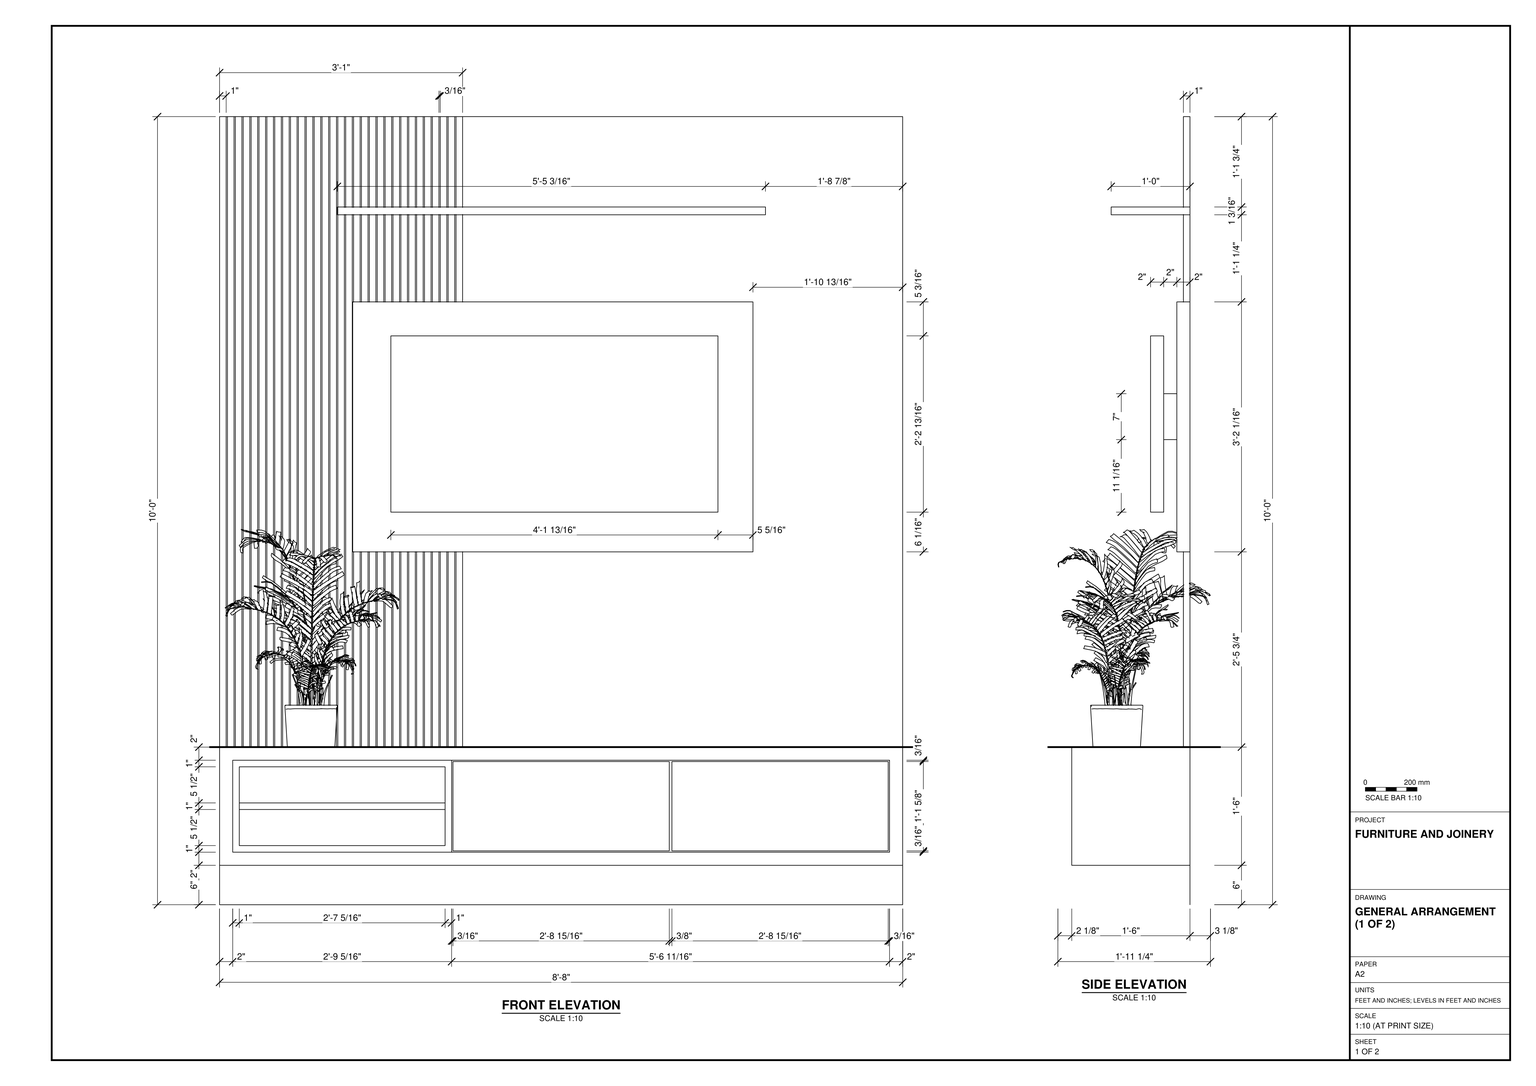
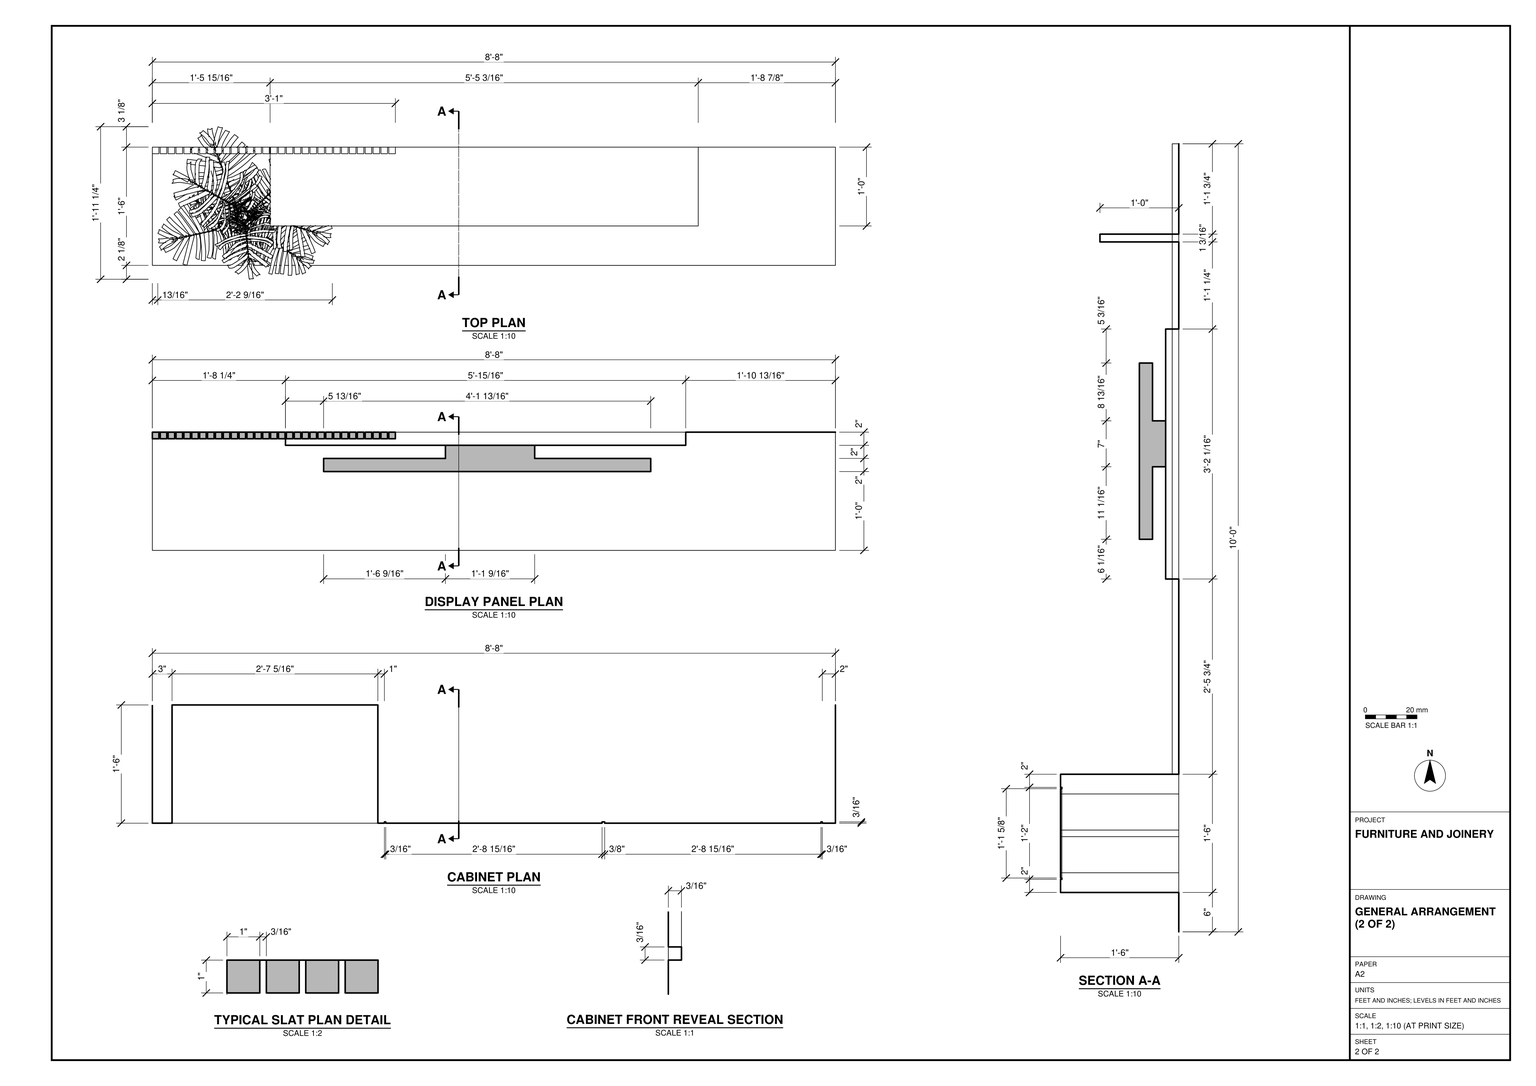
Build the display wall in SketchUp from task_files/diagram_01.pdf. Work in feet and inches, using the finished floor at ±0'-0" as the datum. The complete arrangement measures 8'-8" wide, 1'-11 1/4" deep and 10'-0" high. Use the cabinet plan and section for the cabinet depth rather than extending it to the overall depth.

Run the cabinet across the full width, with its underside 6" above the floor. Divide the left bay horizontally into two open compartments. Fit the two adjacent fronts to its right, leaving the narrow reveals shown in the details. Above the cabinet, form the left-hand field with evenly spaced vertical slats and leave the right-hand field plain. Place the rectangular backing panel across the transition between the fields. Mount the smaller display forward of the panel on the short central support shown in section. Set the narrow horizontal shelf above the display, with its ends offset from the ends of the cabinet as dimensioned in plan.

Place a potted plant on the left end of the cabinet. Decor and loose items such as the plant may be any suitable library component, for example from 3D Warehouse. Keep distinct joinery pieces in separate groups or components and use components for repeated parts. Save one SketchUp model as output_files/slatted_display_wall_with_a_floating_cabinet.skp.

# SketchUp Ruby script. Lengths in inches.
U = 1.inch
M = Sketchup.active_model
def pt(a) = Geom::Point3d.new(a.map { |v| v * U })
def face(e, loops, mat)
  f = e.add_face(loops[0].map { |a| pt(a) })
  loops[1..].each { |l| e.add_face(l.map { |a| pt(a) }).erase! }
  f.material = f.back_material = mat if mat
  f
end
# faces: each face lists its corners as indices into pts; further lists are holes
def faces(e, pts, list, mat = nil) = list.each { |f| face(e, (f[0].is_a?(Array) ? f : [f]).map { |l| l.map { |i| pts[i] } }, mat) }
# xy, xz, yz: faces in a plane at the given z, y or x. An outline is a flat list of corners, or four numbers for a rectangle; further outlines are holes
def ring(l) = l.size == 4 ? [[l[0], l[1]], [l[2], l[1]], [l[2], l[3]], [l[0], l[3]]] : l.each_slice(2).to_a
def flat(e, list, mat, &to3) = list.each { |f| face(e, (f[0].is_a?(Array) ? f : [f]).map { |l| ring(l).map { |u, v| to3.(u, v) } }, mat) }
def xy(e, z, list, mat = nil) = flat(e, list, mat) { |x, y| [x, y, z] }
def xz(e, y, list, mat = nil) = flat(e, list, mat) { |x, z| [x, y, z] }
def yz(e, x, list, mat = nil) = flat(e, list, mat) { |y, z| [x, y, z] }
def lines(e, pts, list) = list.each { |a, b| e.add_line(pt(pts[a]), pt(pts[b])) }
# prism: a flat outline (further loops are holes) pulled along v
def prism(e, loops, v, mat = nil)
  f = face(e, loops, mat); d = Geom::Vector3d.new(v.map { |x| x * U })
  f.pushpull(f.normal.samedirection?(d) ? d.length : -d.length)
end
def box(e, o, s, mat = nil) = prism(e, [[o, [o[0] + s[0], o[1], o[2]], [o[0] + s[0], o[1] + s[1], o[2]], [o[0], o[1] + s[1], o[2]]]], [0, 0, s[2]], mat)
def at(x, y, z, deg = 0) = Geom::Transformation.translation(pt([x, y, z])) * Geom::Transformation.rotation(ORIGIN, Z_AXIS, deg.degrees)
def axes(o, x, y, z) = Geom::Transformation.new([*x, 0, *y, 0, *z, 0, *pt(o).to_a, 1])
def part(name) = M.definitions.add(name)
# library, detail: a bought-in or finely detailed component or shape, given as its bounding box
def library(name, o, s) = part(name).tap { |d| box(d.entities, o, s) }
def detail(e, o, s) = box(e.add_group.entities, o, s)
def put(e, d, t, mat = nil) = e.add_instance(d, t).tap { |i| i.material = mat if mat }
def group(e, t, mat = nil) = e.add_group.tap { |g| g.transformation = t; g.material = mat if mat }.entities
root = M.entities
M.materials.add("[0137_Black]").color = [0, 0, 0]
c1 = part("Vertical wall slat")
box(c1.entities,[0,-1,0],[1,1,96])
c2 = library("SKT_Nearly Natural 5' Kentia Palm Silk Tree",[-23.18,-17.61,0],[47.48,43.95,59.125])
xy(root,6,[[0,0,104,18]])
xy(root,8,[[35.33,0,102,0.2]])
xy(root,8.2,[[35.53,0,68.47,0.2],[68.87,0,101.8,0.2]])
xy(root,9,[[3,0,34.33,18]])
xy(root,14.5,[[3,0,34.33,18]])
xy(root,15.5,[[3,0,34.33,18]])
xy(root,21,[[3,0,34.33,18]])
xy(root,21.8,[[35.53,0,68.47,0.2],[68.87,0,101.8,0.2]])
xy(root,22,[[35.33,0,102,0.2]])
xy(root,24,[[0,0,104,18]])
xy(root,53.73,[[20.27,16,81.21,18]])
xy(root,91.79,[[20.27,16,81.21,18]])
xy(root,105.05,[[17.93,6,83.11,18]])
xy(root,106.24,[[17.93,6,83.11,18]])
xz(root,0,[[[0,6,104,24],[2,8,102,22]],[[2,8,35.33,22],[3,9,34.33,21]],[35.53,8.2,68.47,21.8],[68.87,8.2,101.8,21.8],[3,14.5,34.33,15.5]])
xz(root,0.2,[[[35.33,8,102,22],[35.53,8.2,68.47,21.8],[68.87,8.2,101.8,21.8]]])
xz(root,6,[[17.93,105.05,83.11,106.24]])
xz(root,16,[[20.27,53.73,81.21,91.79]])
xz(root,18,[[0,0,104,6],[3,9,34.33,14.5],[3,15.5,34.33,21],[[1,24,104,120],[20.27,53.73,81.21,91.79],[17.93,105.05,83.11,106.24]]])
yz(root,0,[[0,6,18,24]])
yz(root,3,[[0,9,18,14.5],[0,15.5,18,21]])
yz(root,17.93,[[6,105.05,18,106.24]])
yz(root,20.27,[[16,53.73,18,91.79]])
yz(root,34.33,[[0,9,18,14.5],[0,15.5,18,21]])
yz(root,35.33,[[0,8,0.2,22]])
yz(root,35.53,[[0,8.2,0.2,21.8]])
yz(root,68.47,[[0,8.2,0.2,21.8]])
yz(root,68.87,[[0,8.2,0.2,21.8]])
yz(root,81.21,[[16,53.73,18,91.79]])
yz(root,83.11,[[6,105.05,18,106.24]])
yz(root,101.8,[[0,8.2,0.2,21.8]])
yz(root,102,[[0,8,0.2,22]])
yz(root,104,[[0,6,18,24]])
put(root,c1,at(0,18,24))
put(root,c1,at(1.2,18,24))
put(root,c1,at(2.4,18,24))
put(root,c1,at(3.6,18,24))
put(root,c1,at(4.8,18,24))
put(root,c1,at(6,18,24))
put(root,c1,at(7.2,18,24))
put(root,c1,at(8.4,18,24))
put(root,c1,at(9.6,18,24))
put(root,c1,at(10.8,18,24))
put(root,c1,at(12,18,24))
put(root,c1,at(13.2,18,24))
put(root,c1,at(14.4,18,24))
put(root,c1,at(15.6,18,24))
put(root,c1,at(16.8,18,24))
put(root,c1,at(18,18,24))
put(root,c1,at(19.2,18,24))
put(root,c1,at(20.4,18,24))
put(root,c1,at(21.6,18,24))
put(root,c1,at(22.8,18,24))
put(root,c1,at(24,18,24))
put(root,c1,at(25.2,18,24))
put(root,c1,at(26.4,18,24))
put(root,c1,at(27.6,18,24))
put(root,c1,at(28.8,18,24))
put(root,c1,at(30,18,24))
put(root,c1,at(31.2,18,24))
put(root,c1,at(32.4,18,24))
put(root,c1,at(33.6,18,24))
put(root,c1,at(34.8,18,24))
put(root,c1,at(36,18,24))
put(root,c2,axes([13.91,6.77,23.33],[0.61,0,0],[0,0.61,0],[0,0,0.61]))
g1 = group(root,at(75.88,12,59.78),"[0137_Black]")
xy(g1,0,[[-49.8,0,0,2]])
xy(g1,11.04,[[-31.25,2,-17.67,4]])
xy(g1,18.03,[[-31.25,2,-17.67,4]])
xy(g1,26.84,[[-49.8,0,0,2]])
xz(g1,0,[[-49.8,0,0,26.84]])
xz(g1,2,[[[-49.8,0,0,26.84],[-31.25,11.04,-17.67,18.03]]])
xz(g1,4,[[-31.25,11.04,-17.67,18.03]])
yz(g1,-49.8,[[0,0,2,26.84]])
yz(g1,-31.25,[[2,11.04,4,18.03]])
yz(g1,-17.67,[[2,11.04,4,18.03]])
yz(g1,0,[[0,0,2,26.84]])
